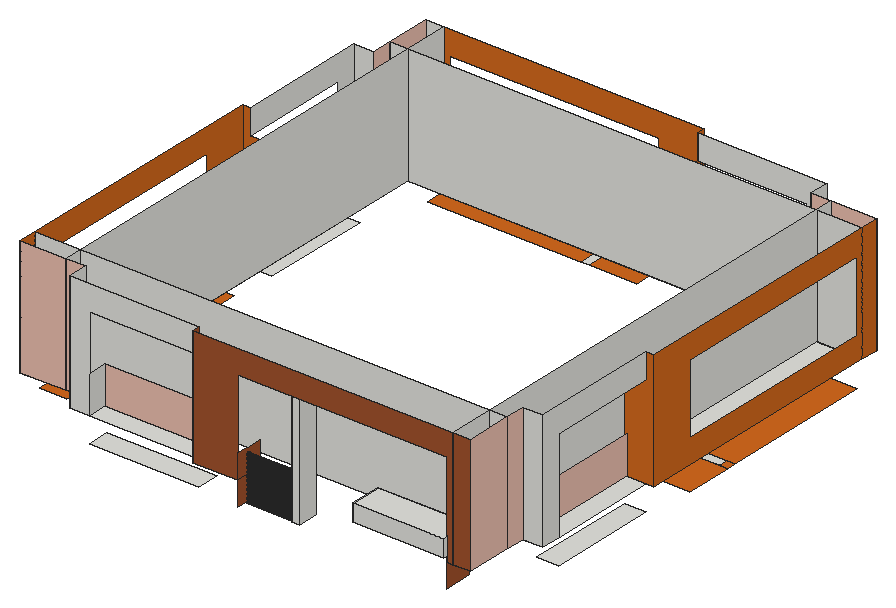
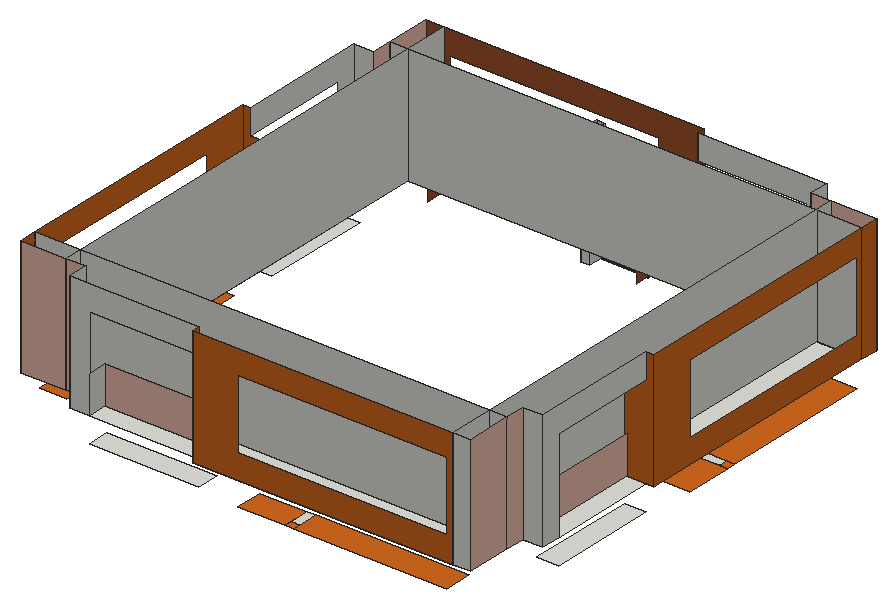
# SketchUp Ruby script. Lengths in inches.
U = 1.inch
M = Sketchup.active_model
def pt(a) = Geom::Point3d.new(a.map { |v| v * U })
def face(e, loops, mat)
  f = e.add_face(loops[0].map { |a| pt(a) })
  loops[1..].each { |l| e.add_face(l.map { |a| pt(a) }).erase! }
  f.material = f.back_material = mat if mat
  f
end
# faces: each face lists its corners as indices into pts; further lists are holes
def faces(e, pts, list, mat = nil) = list.each { |f| face(e, (f[0].is_a?(Array) ? f : [f]).map { |l| l.map { |i| pts[i] } }, mat) }
# xy, xz, yz: faces in a plane at the given z, y or x. An outline is a flat list of corners, or four numbers for a rectangle; further outlines are holes
def ring(l) = l.size == 4 ? [[l[0], l[1]], [l[2], l[1]], [l[2], l[3]], [l[0], l[3]]] : l.each_slice(2).to_a
def flat(e, list, mat, &to3) = list.each { |f| face(e, (f[0].is_a?(Array) ? f : [f]).map { |l| ring(l).map { |u, v| to3.(u, v) } }, mat) }
def xy(e, z, list, mat = nil) = flat(e, list, mat) { |x, y| [x, y, z] }
def xz(e, y, list, mat = nil) = flat(e, list, mat) { |x, z| [x, y, z] }
def yz(e, x, list, mat = nil) = flat(e, list, mat) { |y, z| [x, y, z] }
def lines(e, pts, list) = list.each { |a, b| e.add_line(pt(pts[a]), pt(pts[b])) }
# prism: a flat outline (further loops are holes) pulled along v
def prism(e, loops, v, mat = nil)
  f = face(e, loops, mat); d = Geom::Vector3d.new(v.map { |x| x * U })
  f.pushpull(f.normal.samedirection?(d) ? d.length : -d.length)
end
def box(e, o, s, mat = nil) = prism(e, [[o, [o[0] + s[0], o[1], o[2]], [o[0] + s[0], o[1] + s[1], o[2]], [o[0], o[1] + s[1], o[2]]]], [0, 0, s[2]], mat)
def at(x, y, z, deg = 0) = Geom::Transformation.translation(pt([x, y, z])) * Geom::Transformation.rotation(ORIGIN, Z_AXIS, deg.degrees)
def axes(o, x, y, z) = Geom::Transformation.new([*x, 0, *y, 0, *z, 0, *pt(o).to_a, 1])
def part(name) = M.definitions.add(name)
# library, detail: a bought-in or finely detailed component or shape, given as its bounding box
def library(name, o, s) = part(name).tap { |d| box(d.entities, o, s) }
def detail(e, o, s) = box(e.add_group.entities, o, s)
def put(e, d, t, mat = nil) = e.add_instance(d, t).tap { |i| i.material = mat if mat }
def group(e, t, mat = nil) = e.add_group.tap { |g| g.transformation = t; g.material = mat if mat }.entities
root = M.entities
M.materials.add("[0041_Chocolate]").color = [210, 105, 30]
M.materials.add("[0042_Sienna]").color = [160, 82, 45]
M.materials.add("[0119_RosyBrown]").color = [234, 190, 174]
prism(root,[[[1139,96.8125,1516.98],[1414.89,97.68,1516.98],[1415.2,0.87,1516.98],[1139.3,0,1516.98]]],[0,0,52.19])
xy(root,1422.625,[[306.65,36.8125,641.22,102.8125],[1482,271.47,1548,606.03],[72,943.59,138,1278.16],[978.78,1446.8125,1313.35,1512.8125]])
xy(root,1426.89,[[72,636.29,132,662.8],[1488,886.83,1548,913.33],[671.48,1452.8125,697.99,1512.8125]])
xy(root,1426.89,[[48,169.92,132,636.29],[48,636.29,72,662.8],[48,662.8,132,806.17],[1488,743.45,1572,886.83],[1548,886.83,1572,913.33],
  [1488,913.33,1572,1379.7],[205.11,1452.8125,671.48,1536.8125],[697.99,1452.8125,841.36,1536.8125],[671.48,1512.8125,697.99,1536.8125]],"[0041_Chocolate]")
xy(root,1500,[[1434.3125,12.8125,1488,150.5],[306.65,36.8125,641.22,96.8125],[48,96.8125,185.6875,150.5],[48,150.5,185.6875,150.5,185.6875,1399.125,132,1399.125,132,1338.16,72,1338.16,72,1278.16,132,1278.16,132,943.59,48,943.59],[1434.3125,150.5,1488,150.5,1488,211.46,1548,211.46,1548,271.47,1488,271.47,1488,606.03,1572,606.03,1572,1399.125,1434.3125,1399.125],
  [1488,271.47,1548,606.03],[72,943.59,132,1278.16],[132,1399.125,185.6875,1536.8125],[185.6875,1399.125,1434.3125,1399.125,1434.3125,1452.8125,1373.35,1452.8125,1373.35,1512.8125,1313.35,1512.8125,1313.35,1452.8125,978.78,1452.8125,978.78,1536.8125,185.6875,1536.8125],[1434.3125,1399.125,1572,1452.8125],
  [978.78,1452.8125,1313.35,1512.8125]])
xz(root,12.8125,[[641.22,1500,778.64,1500,778.64,1786.89,1414.89,1786.89,1414.89,1500,1434.3125,1500,1434.3125,1860,641.22,1860],[1434.3125,1500,1488,1860]],"[0042_Sienna]")
xz(root,36.8125,[[922.01,1426.89,948.52,1786.89],[246.65,1500,306.65,1500,306.65,1782.625,641.22,1782.625,641.22,1860,246.65,1860]])
xz(root,96.8125,[[922.01,1426.89,948.52,1786.89]])
xz(root,96.8125,[[48,1500,185.6875,1860],[185.6875,1500,246.65,1860],[306.65,1500,641.22,1613.76]],"[0119_RosyBrown]")
xz(root,150.5,[[48,1500,1488,1860]])
xz(root,211.46,[[1488,1500,1548,1860]])
xz(root,271.47,[[1488,1500,1548,1613.76]])
xz(root,606.03,[[1488,1500,1572,1500,1572,1860,1548,1860,1548,1782.625,1482,1782.625,1482,1613.76,1488,1613.76]],"[0041_Chocolate]")
xz(root,943.59,[[48,1500,48,1860,72,1860,72,1782.625,138,1782.625,138,1613.76,132,1613.76,132,1500]],"[0041_Chocolate]")
xz(root,1278.16,[[72,1500,132,1613.76]])
xz(root,1338.16,[[72,1500,132,1860]])
xz(root,1399.125,[[132,1500,1572,1860]])
xz(root,1452.8125,[[978.78,1500,1313.35,1613.76],[1373.35,1500,1434.3125,1860],[1434.3125,1500,1572,1860]],"[0119_RosyBrown]")
xz(root,1512.8125,[[1313.35,1500,1313.35,1782.625,978.78,1782.625,978.78,1860,1373.35,1860,1373.35,1500]])
xz(root,1536.8125,[[132,1500,185.6875,1860]])
xz(root,1536.8125,[[[185.6875,1500,978.78,1860],[205.11,1573.11,841.36,1786.89]]],"[0041_Chocolate]")
yz(root,48,[[96.8125,1500,150.5,1860],[[150.5,1500,943.59,1860],[169.92,1573.11,806.17,1786.89]]],"[0041_Chocolate]")
yz(root,72,[[1278.16,1500,1278.16,1782.625,943.59,1782.625,943.59,1860,1338.16,1860,1338.16,1500]])
yz(root,132,[[943.59,1500,1278.16,1613.76],[1338.16,1500,1399.125,1860],[1399.125,1500,1536.8125,1860]],"[0119_RosyBrown]")
yz(root,185.6875,[[96.8125,1500,1536.8125,1860]])
yz(root,246.65,[[36.8125,1500,96.8125,1860]])
yz(root,306.65,[[36.8125,1500,96.8125,1613.76]])
yz(root,641.22,[[12.8125,1500,12.8125,1860,36.8125,1860,36.8125,1782.625,102.8125,1782.625,102.8125,1613.76,96.8125,1613.76,96.8125,1500]],"[0042_Sienna]")
yz(root,778.64,[[48.34,1422.02,49.29,1422.14,50.18,1422.51,50.95,1423.1,51.53,1423.86,51.9,1424.75,52.03,1425.7,51.9,1426.66,51.8,1426.89,44.875,1426.89,44.78,1426.66,44.65,1425.7,44.78,1424.75,45.15,1423.86,45.73,1423.1,46.5,1422.51,47.38,1422.14]])
yz(root,778.64,[[12.8125,1426.89,44.875,1426.89,45.15,1427.55,45.73,1428.3125,46.5,1428.9,47.38,1429.27,48.34,1429.39,49.29,1429.27,50.18,1428.9,50.95,1428.3125,51.53,1427.55,51.8,1426.89,96.8125,1426.89,96.8125,1500,51.19,1500,51.53,1499.55,51.9,1498.66,52.03,1497.7,51.9,1496.75,51.53,1495.86,50.95,1495.1,50.18,1494.51,49.29,1494.14,48.34,1494.02,47.38,1494.14,46.5,1494.51,45.73,1495.1,45.15,1495.86,44.78,1496.75,44.65,1497.7,44.78,1498.66,45.15,1499.55,45.49,1500,12.8125,1500],[44.875,1426.89,51.8,1426.89,51.53,1427.55,50.95,1428.3125,50.18,1428.9,49.29,1429.27,48.34,1429.39,47.38,1429.27,46.5,1428.9,45.73,1428.3125,45.15,1427.55],[48.34,1494.02,49.29,1494.14,50.18,1494.51,50.95,1495.1,51.53,1495.86,51.9,1496.75,52.03,1497.7,51.9,1498.66,51.53,1499.55,51.19,1500,45.49,1500,45.15,1499.55,44.78,1498.66,44.65,1497.7,44.78,1496.75,45.15,1495.86,45.73,1495.1,46.5,1494.51,47.38,1494.14],[12.8125,1500,45.49,1500,45.73,1500.3125,46.5,1500.9,47.38,1501.27,48.34,1501.39,49.29,1501.27,50.18,1500.9,50.95,1500.3125,51.19,1500,96.8125,1500,96.8125,1573.11,49.67,1573.11,50.18,1572.9,50.95,1572.3125,51.53,1571.55,51.9,1570.66,52.03,1569.7,51.9,1568.75,51.53,1567.86,50.95,1567.1,50.18,1566.51,49.29,1566.14,48.34,1566.02,47.38,1566.14,46.5,1566.51,45.73,1567.1,45.15,1567.86,44.78,1568.75,44.65,1569.7,44.78,1570.66,45.15,1571.55,45.73,1572.3125,46.5,1572.9,47.01,1573.11,12.8125,1573.11],[45.49,1500,51.19,1500,50.95,1500.3125,50.18,1500.9,49.29,1501.27,48.34,1501.39,47.38,1501.27,46.5,1500.9,45.73,1500.3125]],"[0042_Sienna]")
yz(root,922.01,[[48.34,1422.02,47.38,1422.14,46.5,1422.51,45.73,1423.1,45.15,1423.86,44.78,1424.75,44.65,1425.7,44.78,1426.66,44.875,1426.89,51.8,1426.89,51.9,1426.66,52.03,1425.7,51.9,1424.75,51.53,1423.86,50.95,1423.1,50.18,1422.51,49.29,1422.14],[[36.8125,1426.89,36.8125,1786.89,96.8125,1786.89,96.8125,1426.89,51.8,1426.89,51.53,1427.55,50.95,1428.3125,50.18,1428.9,49.29,1429.27,48.34,1429.39,47.38,1429.27,46.5,1428.9,45.73,1428.3125,45.15,1427.55,44.875,1426.89],[48.34,1578.02,49.29,1578.14,50.18,1578.51,50.95,1579.1,51.53,1579.86,51.9,1580.75,52.03,1581.7,51.9,1582.66,51.53,1583.55,50.95,1584.3125,50.18,1584.9,49.29,1585.27,48.34,1585.39,47.38,1585.27,46.5,1584.9,45.73,1584.3125,45.15,1583.55,44.78,1582.66,44.65,1581.7,44.78,1580.75,45.15,1579.86,45.73,1579.1,46.5,1578.51,47.38,1578.14]],[44.875,1426.89,45.15,1427.55,45.73,1428.3125,46.5,1428.9,47.38,1429.27,48.34,1429.39,49.29,1429.27,50.18,1428.9,50.95,1428.3125,51.53,1427.55,51.8,1426.89]])
yz(root,948.52,[[36.8125,1426.89,96.8125,1786.89]])
yz(root,978.78,[[1452.8125,1500,1536.8125,1500,1536.8125,1860,1512.8125,1860,1512.8125,1782.625,1446.8125,1782.625,1446.8125,1613.76,1452.8125,1613.76]],"[0041_Chocolate]")
yz(root,1313.35,[[1452.8125,1500,1512.8125,1613.76]])
yz(root,1373.35,[[1452.8125,1500,1512.8125,1860]])
yz(root,1414.89,[[12.8125,1426.89,96.8125,1500],[12.8125,1500,96.8125,1573.11]],"[0042_Sienna]")
yz(root,1434.3125,[[12.8125,1500,1452.8125,1860]])
yz(root,1488,[[12.8125,1500,150.5,1860],[150.5,1500,211.46,1860],[271.47,1500,606.03,1613.76]],"[0119_RosyBrown]")
yz(root,1548,[[211.46,1500,271.47,1500,271.47,1782.625,606.03,1782.625,606.03,1860,211.46,1860]])
yz(root,1572,[[[606.03,1500,1399.125,1860],[743.45,1573.11,1379.7,1786.89]],[1399.125,1500,1452.8125,1860]],"[0041_Chocolate]")
p = [[922.01,48.34,1422.02],[922.01,47.38,1422.14],[778.64,47.38,1422.14],[778.64,48.34,1422.02],[922.01,49.29,1422.14],[778.64,49.29,1422.14],
  [922.01,46.5,1422.51],[778.64,46.5,1422.51],[922.01,50.18,1422.51],[778.64,50.18,1422.51],[922.01,45.73,1423.1],[778.64,45.73,1423.1],
  [922.01,50.95,1423.1],[778.64,50.95,1423.1],[922.01,45.15,1423.86],[778.64,45.15,1423.86],[922.01,51.53,1423.86],[778.64,51.53,1423.86],
  [922.01,44.78,1424.75],[778.64,44.78,1424.75],[922.01,51.9,1424.75],[778.64,51.9,1424.75],[922.01,44.65,1425.7],[778.64,44.65,1425.7],
  [922.01,52.03,1425.7],[778.64,52.03,1425.7],[922.01,44.78,1426.66],[778.64,44.78,1426.66],[922.01,51.9,1426.66],[778.64,51.9,1426.66],
  [922.01,44.875,1426.89],[922.01,45.15,1427.55],[778.64,45.15,1427.55],[778.64,44.875,1426.89],[922.01,51.53,1427.55],[922.01,51.8,1426.89],
  [778.64,51.8,1426.89],[778.64,51.53,1427.55],[922.01,45.73,1428.3125],[778.64,45.73,1428.3125],[922.01,50.95,1428.3125],[778.64,50.95,1428.3125],
  [922.01,46.5,1428.9],[778.64,46.5,1428.9],[922.01,50.18,1428.9],[778.64,50.18,1428.9],[922.01,47.38,1429.27],[778.64,47.38,1429.27],
  [922.01,49.29,1429.27],[778.64,49.29,1429.27],[922.01,48.34,1429.39],[778.64,48.34,1429.39],[922.01,48.34,1434.02],[922.01,47.38,1434.14],
  [778.64,47.38,1434.14],[778.64,48.34,1434.02],[922.01,49.29,1434.14],[778.64,49.29,1434.14],[922.01,46.5,1434.51],[778.64,46.5,1434.51],
  [922.01,50.18,1434.51],[778.64,50.18,1434.51],[922.01,45.73,1435.1],[778.64,45.73,1435.1],[922.01,50.95,1435.1],[778.64,50.95,1435.1],
  [922.01,45.15,1435.86],[778.64,45.15,1435.86],[922.01,51.53,1435.86],[778.64,51.53,1435.86],[922.01,44.78,1436.75],[778.64,44.78,1436.75],
  [922.01,51.9,1436.75],[778.64,51.9,1436.75],[922.01,44.65,1437.7],[778.64,44.65,1437.7],[922.01,52.03,1437.7],[778.64,52.03,1437.7],
  [922.01,44.78,1438.66],[778.64,44.78,1438.66],[922.01,51.9,1438.66],[778.64,51.9,1438.66],[922.01,45.15,1439.55],[778.64,45.15,1439.55],
  [922.01,51.53,1439.55],[778.64,51.53,1439.55],[922.01,45.73,1440.3125],[778.64,45.73,1440.3125],[922.01,50.95,1440.3125],[778.64,50.95,1440.3125],
  [922.01,46.5,1440.9],[778.64,46.5,1440.9],[922.01,50.18,1440.9],[778.64,50.18,1440.9],[922.01,47.38,1441.27],[778.64,47.38,1441.27],
  [922.01,49.29,1441.27],[778.64,49.29,1441.27],[922.01,48.34,1441.39],[778.64,48.34,1441.39],[922.01,48.34,1446.02],[922.01,47.38,1446.14],
  [778.64,47.38,1446.14],[778.64,48.34,1446.02],[922.01,49.29,1446.14],[778.64,49.29,1446.14],[922.01,46.5,1446.51],[778.64,46.5,1446.51],
  [922.01,50.18,1446.51],[778.64,50.18,1446.51],[922.01,45.73,1447.1],[778.64,45.73,1447.1],[922.01,50.95,1447.1],[778.64,50.95,1447.1],
  [922.01,45.15,1447.86],[778.64,45.15,1447.86],[922.01,51.53,1447.86],[778.64,51.53,1447.86],[922.01,44.78,1448.75],[778.64,44.78,1448.75],
  [922.01,51.9,1448.75],[778.64,51.9,1448.75],[922.01,44.65,1449.7],[778.64,44.65,1449.7],[922.01,52.03,1449.7],[778.64,52.03,1449.7],
  [922.01,44.78,1450.66],[778.64,44.78,1450.66],[922.01,51.9,1450.66],[778.64,51.9,1450.66],[922.01,45.15,1451.55],[778.64,45.15,1451.55],
  [922.01,51.53,1451.55],[778.64,51.53,1451.55],[922.01,45.73,1452.3125],[778.64,45.73,1452.3125],[922.01,50.95,1452.3125],[778.64,50.95,1452.3125],
  [922.01,46.5,1452.9],[778.64,46.5,1452.9],[922.01,50.18,1452.9],[778.64,50.18,1452.9],[922.01,47.38,1453.27],[778.64,47.38,1453.27],
  [922.01,49.29,1453.27],[778.64,49.29,1453.27],[922.01,48.34,1453.39],[778.64,48.34,1453.39],[922.01,48.34,1458.02],[922.01,47.38,1458.14],
  [778.64,47.38,1458.14],[778.64,48.34,1458.02],[922.01,49.29,1458.14],[778.64,49.29,1458.14],[922.01,46.5,1458.51],[778.64,46.5,1458.51],
  [922.01,50.18,1458.51],[778.64,50.18,1458.51],[922.01,45.73,1459.1],[778.64,45.73,1459.1],[922.01,50.95,1459.1],[778.64,50.95,1459.1],
  [922.01,45.15,1459.86],[778.64,45.15,1459.86],[922.01,51.53,1459.86],[778.64,51.53,1459.86],[922.01,44.78,1460.75],[778.64,44.78,1460.75],
  [922.01,51.9,1460.75],[778.64,51.9,1460.75],[922.01,44.65,1461.7],[778.64,44.65,1461.7],[922.01,52.03,1461.7],[778.64,52.03,1461.7],
  [922.01,44.78,1462.66],[778.64,44.78,1462.66],[922.01,51.9,1462.66],[778.64,51.9,1462.66],[922.01,45.15,1463.55],[778.64,45.15,1463.55],
  [922.01,51.53,1463.55],[778.64,51.53,1463.55],[922.01,45.73,1464.3125],[778.64,45.73,1464.3125],[922.01,50.95,1464.3125],[778.64,50.95,1464.3125],
  [922.01,46.5,1464.9],[778.64,46.5,1464.9],[922.01,50.18,1464.9],[778.64,50.18,1464.9],[922.01,47.38,1465.27],[778.64,47.38,1465.27],
  [922.01,49.29,1465.27],[778.64,49.29,1465.27],[922.01,48.34,1465.39],[778.64,48.34,1465.39],[922.01,48.34,1470.02],[922.01,47.38,1470.14],
  [778.64,47.38,1470.14],[778.64,48.34,1470.02],[922.01,49.29,1470.14],[778.64,49.29,1470.14],[922.01,46.5,1470.51],[778.64,46.5,1470.51],
  [922.01,50.18,1470.51],[778.64,50.18,1470.51],[922.01,45.73,1471.1],[778.64,45.73,1471.1],[922.01,50.95,1471.1],[778.64,50.95,1471.1],
  [922.01,45.15,1471.86],[778.64,45.15,1471.86],[922.01,51.53,1471.86],[778.64,51.53,1471.86],[922.01,44.78,1472.75],[778.64,44.78,1472.75],
  [922.01,51.9,1472.75],[778.64,51.9,1472.75],[922.01,44.65,1473.7],[778.64,44.65,1473.7],[922.01,52.03,1473.7],[778.64,52.03,1473.7],
  [922.01,44.78,1474.66],[778.64,44.78,1474.66],[922.01,51.9,1474.66],[778.64,51.9,1474.66],[922.01,45.15,1475.55],[778.64,45.15,1475.55],
  [922.01,51.53,1475.55],[778.64,51.53,1475.55],[922.01,45.73,1476.3125],[778.64,45.73,1476.3125],[922.01,50.95,1476.3125],[778.64,50.95,1476.3125],
  [922.01,46.5,1476.9],[778.64,46.5,1476.9],[922.01,50.18,1476.9],[778.64,50.18,1476.9],[922.01,47.38,1477.27],[778.64,47.38,1477.27],
  [922.01,49.29,1477.27],[778.64,49.29,1477.27],[922.01,48.34,1477.39],[778.64,48.34,1477.39],[922.01,48.34,1482.02],[922.01,47.38,1482.14],
  [778.64,47.38,1482.14],[778.64,48.34,1482.02],[922.01,49.29,1482.14],[778.64,49.29,1482.14],[922.01,46.5,1482.51],[778.64,46.5,1482.51],
  [922.01,50.18,1482.51],[778.64,50.18,1482.51],[922.01,45.73,1483.1],[778.64,45.73,1483.1],[922.01,50.95,1483.1],[778.64,50.95,1483.1],
  [922.01,45.15,1483.86],[778.64,45.15,1483.86],[922.01,51.53,1483.86],[778.64,51.53,1483.86],[922.01,44.78,1484.75],[778.64,44.78,1484.75],
  [922.01,51.9,1484.75],[778.64,51.9,1484.75],[922.01,44.65,1485.7],[778.64,44.65,1485.7],[922.01,52.03,1485.7],[778.64,52.03,1485.7],
  [922.01,44.78,1486.66],[778.64,44.78,1486.66],[922.01,51.9,1486.66],[778.64,51.9,1486.66],[922.01,45.15,1487.55],[778.64,45.15,1487.55],
  [922.01,51.53,1487.55],[778.64,51.53,1487.55],[922.01,45.73,1488.3125],[778.64,45.73,1488.3125],[922.01,50.95,1488.3125],[778.64,50.95,1488.3125],
  [922.01,46.5,1488.9],[778.64,46.5,1488.9],[922.01,50.18,1488.9],[778.64,50.18,1488.9],[922.01,47.38,1489.27],[778.64,47.38,1489.27],
  [922.01,49.29,1489.27],[778.64,49.29,1489.27],[922.01,48.34,1489.39],[778.64,48.34,1489.39],[922.01,48.34,1494.02],[922.01,47.38,1494.14],
  [778.64,47.38,1494.14],[778.64,48.34,1494.02],[922.01,49.29,1494.14],[778.64,49.29,1494.14],[922.01,46.5,1494.51],[778.64,46.5,1494.51],
  [922.01,50.18,1494.51],[778.64,50.18,1494.51],[922.01,45.73,1495.1],[778.64,45.73,1495.1],[922.01,50.95,1495.1],[778.64,50.95,1495.1],
  [922.01,45.15,1495.86],[778.64,45.15,1495.86],[922.01,51.53,1495.86],[778.64,51.53,1495.86],[922.01,44.78,1496.75],[778.64,44.78,1496.75],
  [922.01,51.9,1496.75],[778.64,51.9,1496.75],[922.01,44.65,1497.7],[778.64,44.65,1497.7],[922.01,52.03,1497.7],[778.64,52.03,1497.7],
  [922.01,44.78,1498.66],[778.64,44.78,1498.66],[922.01,51.9,1498.66],[778.64,51.9,1498.66],[922.01,45.15,1499.55],[778.64,45.15,1499.55],
  [922.01,51.53,1499.55],[778.64,51.53,1499.55],[922.01,45.73,1500.3125],[778.64,45.73,1500.3125],[778.64,45.49,1500],[922.01,50.95,1500.3125],
  [778.64,51.19,1500],[778.64,50.95,1500.3125],[922.01,46.5,1500.9],[778.64,46.5,1500.9],[922.01,50.18,1500.9],[778.64,50.18,1500.9],
  [922.01,47.38,1501.27],[778.64,47.38,1501.27],[922.01,49.29,1501.27],[778.64,49.29,1501.27],[922.01,48.34,1501.39],[778.64,48.34,1501.39],
  [922.01,48.34,1506.02],[922.01,47.38,1506.14],[778.64,47.38,1506.14],[778.64,48.34,1506.02],[922.01,49.29,1506.14],[778.64,49.29,1506.14],
  [922.01,46.5,1506.51],[778.64,46.5,1506.51],[922.01,50.18,1506.51],[778.64,50.18,1506.51],[922.01,45.73,1507.1],[778.64,45.73,1507.1],
  [922.01,50.95,1507.1],[778.64,50.95,1507.1],[922.01,45.15,1507.86],[778.64,45.15,1507.86],[922.01,51.53,1507.86],[778.64,51.53,1507.86],
  [922.01,44.78,1508.75],[778.64,44.78,1508.75],[922.01,51.9,1508.75],[778.64,51.9,1508.75],[922.01,44.65,1509.7],[778.64,44.65,1509.7],
  [922.01,52.03,1509.7],[778.64,52.03,1509.7],[922.01,44.78,1510.66],[778.64,44.78,1510.66],[922.01,51.9,1510.66],[778.64,51.9,1510.66],
  [922.01,45.15,1511.55],[778.64,45.15,1511.55],[922.01,51.53,1511.55],[778.64,51.53,1511.55],[922.01,45.73,1512.3125],[778.64,45.73,1512.3125],
  [922.01,50.95,1512.3125],[778.64,50.95,1512.3125],[922.01,46.5,1512.9],[778.64,46.5,1512.9],[922.01,50.18,1512.9],[778.64,50.18,1512.9],
  [922.01,47.38,1513.27],[778.64,47.38,1513.27],[922.01,49.29,1513.27],[778.64,49.29,1513.27],[922.01,48.34,1513.39],[778.64,48.34,1513.39],
  [922.01,48.34,1518.02],[922.01,47.38,1518.14],[778.64,47.38,1518.14],[778.64,48.34,1518.02],[922.01,49.29,1518.14],[778.64,49.29,1518.14],
  [922.01,46.5,1518.51],[778.64,46.5,1518.51],[922.01,50.18,1518.51],[778.64,50.18,1518.51],[922.01,45.73,1519.1],[778.64,45.73,1519.1],
  [922.01,50.95,1519.1],[778.64,50.95,1519.1],[922.01,45.15,1519.86],[778.64,45.15,1519.86],[922.01,51.53,1519.86],[778.64,51.53,1519.86],
  [922.01,44.78,1520.75],[778.64,44.78,1520.75],[922.01,51.9,1520.75],[778.64,51.9,1520.75],[922.01,44.65,1521.7],[778.64,44.65,1521.7],
  [922.01,52.03,1521.7],[778.64,52.03,1521.7],[922.01,44.78,1522.66],[778.64,44.78,1522.66],[922.01,51.9,1522.66],[778.64,51.9,1522.66],
  [922.01,45.15,1523.55],[778.64,45.15,1523.55],[922.01,51.53,1523.55],[778.64,51.53,1523.55],[922.01,45.73,1524.3125],[778.64,45.73,1524.3125],
  [922.01,50.95,1524.3125],[778.64,50.95,1524.3125],[922.01,46.5,1524.9],[778.64,46.5,1524.9],[922.01,50.18,1524.9],[778.64,50.18,1524.9],
  [922.01,47.38,1525.27],[778.64,47.38,1525.27],[922.01,49.29,1525.27],[778.64,49.29,1525.27],[922.01,48.34,1525.39],[778.64,48.34,1525.39],
  [922.01,48.34,1530.02],[922.01,47.38,1530.14],[778.64,47.38,1530.14],[778.64,48.34,1530.02],[922.01,49.29,1530.14],[778.64,49.29,1530.14],
  [922.01,46.5,1530.51],[778.64,46.5,1530.51],[922.01,50.18,1530.51],[778.64,50.18,1530.51],[922.01,45.73,1531.1],[778.64,45.73,1531.1],
  [922.01,50.95,1531.1],[778.64,50.95,1531.1],[922.01,45.15,1531.86],[778.64,45.15,1531.86],[922.01,51.53,1531.86],[778.64,51.53,1531.86],
  [922.01,44.78,1532.75],[778.64,44.78,1532.75],[922.01,51.9,1532.75],[778.64,51.9,1532.75],[922.01,44.65,1533.7],[778.64,44.65,1533.7],
  [922.01,52.03,1533.7],[778.64,52.03,1533.7],[922.01,44.78,1534.66],[778.64,44.78,1534.66],[922.01,51.9,1534.66],[778.64,51.9,1534.66],
  [922.01,45.15,1535.55],[778.64,45.15,1535.55],[922.01,51.53,1535.55],[778.64,51.53,1535.55],[922.01,45.73,1536.3125],[778.64,45.73,1536.3125],
  [922.01,50.95,1536.3125],[778.64,50.95,1536.3125],[922.01,46.5,1536.9],[778.64,46.5,1536.9],[922.01,50.18,1536.9],[778.64,50.18,1536.9],
  [922.01,47.38,1537.27],[778.64,47.38,1537.27],[922.01,49.29,1537.27],[778.64,49.29,1537.27],[922.01,48.34,1537.39],[778.64,48.34,1537.39],
  [922.01,48.34,1542.02],[922.01,47.38,1542.14],[778.64,47.38,1542.14],[778.64,48.34,1542.02],[922.01,49.29,1542.14],[778.64,49.29,1542.14],
  [922.01,46.5,1542.51],[778.64,46.5,1542.51],[922.01,50.18,1542.51],[778.64,50.18,1542.51],[922.01,45.73,1543.1],[778.64,45.73,1543.1],
  [922.01,50.95,1543.1],[778.64,50.95,1543.1],[922.01,45.15,1543.86],[778.64,45.15,1543.86],[922.01,51.53,1543.86],[778.64,51.53,1543.86],
  [922.01,44.78,1544.75],[778.64,44.78,1544.75],[922.01,51.9,1544.75],[778.64,51.9,1544.75],[922.01,44.65,1545.7],[778.64,44.65,1545.7],
  [922.01,52.03,1545.7],[778.64,52.03,1545.7],[922.01,44.78,1546.66],[778.64,44.78,1546.66],[922.01,51.9,1546.66],[778.64,51.9,1546.66],
  [922.01,45.15,1547.55],[778.64,45.15,1547.55],[922.01,51.53,1547.55],[778.64,51.53,1547.55],[922.01,45.73,1548.3125],[778.64,45.73,1548.3125],
  [922.01,50.95,1548.3125],[778.64,50.95,1548.3125],[922.01,46.5,1548.9],[778.64,46.5,1548.9],[922.01,50.18,1548.9],[778.64,50.18,1548.9],
  [922.01,47.38,1549.27],[778.64,47.38,1549.27],[922.01,49.29,1549.27],[778.64,49.29,1549.27],[922.01,48.34,1549.39],[778.64,48.34,1549.39],
  [922.01,48.34,1554.02],[922.01,47.38,1554.14],[778.64,47.38,1554.14],[778.64,48.34,1554.02],[922.01,49.29,1554.14],[778.64,49.29,1554.14],
  [922.01,46.5,1554.51],[778.64,46.5,1554.51],[922.01,50.18,1554.51],[778.64,50.18,1554.51],[922.01,45.73,1555.1],[778.64,45.73,1555.1],
  [922.01,50.95,1555.1],[778.64,50.95,1555.1],[922.01,45.15,1555.86],[778.64,45.15,1555.86],[922.01,51.53,1555.86],[778.64,51.53,1555.86],
  [922.01,44.78,1556.75],[778.64,44.78,1556.75],[922.01,51.9,1556.75],[778.64,51.9,1556.75],[922.01,44.65,1557.7],[778.64,44.65,1557.7],
  [922.01,52.03,1557.7],[778.64,52.03,1557.7],[922.01,44.78,1558.66],[778.64,44.78,1558.66],[922.01,51.9,1558.66],[778.64,51.9,1558.66],
  [922.01,45.15,1559.55],[778.64,45.15,1559.55],[922.01,51.53,1559.55],[778.64,51.53,1559.55],[922.01,45.73,1560.3125],[778.64,45.73,1560.3125],
  [922.01,50.95,1560.3125],[778.64,50.95,1560.3125],[922.01,46.5,1560.9],[778.64,46.5,1560.9],[922.01,50.18,1560.9],[778.64,50.18,1560.9],
  [922.01,47.38,1561.27],[778.64,47.38,1561.27],[922.01,49.29,1561.27],[778.64,49.29,1561.27],[922.01,48.34,1561.39],[778.64,48.34,1561.39]]
faces(root,p,[[0,1,2,3],[4,0,3,5],[1,6,7,2],[8,4,5,9],[6,10,11,7],[12,8,9,13],[10,14,15,11],[16,12,13,17],
  [14,18,19,15],[20,16,17,21],[18,22,23,19],[24,20,21,25],[22,26,27,23],[28,24,25,29],[26,30,31,32,33,27],[34,35,28,29,36,37],
  [31,38,39,32],[40,34,37,41],[38,42,43,39],[44,40,41,45],[42,46,47,43],[48,44,45,49],[46,50,51,47],[50,48,49,51],
  [52,53,54,55],[56,52,55,57],[53,58,59,54],[60,56,57,61],[58,62,63,59],[64,60,61,65],[62,66,67,63],[68,64,65,69],
  [66,70,71,67],[72,68,69,73],[70,74,75,71],[76,72,73,77],[74,78,79,75],[80,76,77,81],[78,82,83,79],[84,80,81,85],
  [82,86,87,83],[88,84,85,89],[86,90,91,87],[92,88,89,93],[90,94,95,91],[96,92,93,97],[94,98,99,95],[98,96,97,99],
  [100,101,102,103],[104,100,103,105],[101,106,107,102],[108,104,105,109],[106,110,111,107],[112,108,109,113],[110,114,115,111],[116,112,113,117],
  [114,118,119,115],[120,116,117,121],[118,122,123,119],[124,120,121,125],[122,126,127,123],[128,124,125,129],[126,130,131,127],[132,128,129,133],
  [130,134,135,131],[136,132,133,137],[134,138,139,135],[140,136,137,141],[138,142,143,139],[144,140,141,145],[142,146,147,143],[146,144,145,147],
  [148,149,150,151],[152,148,151,153],[149,154,155,150],[156,152,153,157],[154,158,159,155],[160,156,157,161],[158,162,163,159],[164,160,161,165],
  [162,166,167,163],[168,164,165,169],[166,170,171,167],[172,168,169,173],[170,174,175,171],[176,172,173,177],[174,178,179,175],[180,176,177,181],
  [178,182,183,179],[184,180,181,185],[182,186,187,183],[188,184,185,189],[186,190,191,187],[192,188,189,193],[190,194,195,191],[194,192,193,195],
  [196,197,198,199],[200,196,199,201],[197,202,203,198],[204,200,201,205],[202,206,207,203],[208,204,205,209],[206,210,211,207],[212,208,209,213],
  [210,214,215,211],[216,212,213,217],[214,218,219,215],[220,216,217,221],[218,222,223,219],[224,220,221,225],[222,226,227,223],[228,224,225,229],
  [226,230,231,227],[232,228,229,233],[230,234,235,231],[236,232,233,237],[234,238,239,235],[240,236,237,241],[238,242,243,239],[242,240,241,243],
  [244,245,246,247],[248,244,247,249],[245,250,251,246],[252,248,249,253],[250,254,255,251],[256,252,253,257],[254,258,259,255],[260,256,257,261],
  [258,262,263,259],[264,260,261,265],[262,266,267,263],[268,264,265,269],[266,270,271,267],[272,268,269,273],[270,274,275,271],[276,272,273,277],
  [274,278,279,275],[280,276,277,281],[278,282,283,279],[284,280,281,285],[282,286,287,283],[288,284,285,289],[286,290,291,287],[290,288,289,291],
  [292,293,294,295],[296,292,295,297],[293,298,299,294],[300,296,297,301],[298,302,303,299],[304,300,301,305],[302,306,307,303],[308,304,305,309],
  [306,310,311,307],[312,308,309,313],[310,314,315,311],[316,312,313,317],[314,318,319,315],[320,316,317,321],[318,322,323,319],[324,320,321,325],
  [322,326,327,328,323],[329,324,325,330,331],[326,332,333,327],[334,329,331,335],[332,336,337,333],[338,334,335,339],[336,340,341,337],[340,338,339,341],
  [342,343,344,345],[346,342,345,347],[343,348,349,344],[350,346,347,351],[348,352,353,349],[354,350,351,355],[352,356,357,353],[358,354,355,359],
  [356,360,361,357],[362,358,359,363],[360,364,365,361],[366,362,363,367],[364,368,369,365],[370,366,367,371],[368,372,373,369],[374,370,371,375],
  [372,376,377,373],[378,374,375,379],[376,380,381,377],[382,378,379,383],[380,384,385,381],[386,382,383,387],[384,388,389,385],[388,386,387,389],
  [390,391,392,393],[394,390,393,395],[391,396,397,392],[398,394,395,399],[396,400,401,397],[402,398,399,403],[400,404,405,401],[406,402,403,407],
  [404,408,409,405],[410,406,407,411],[408,412,413,409],[414,410,411,415],[412,416,417,413],[418,414,415,419],[416,420,421,417],[422,418,419,423],
  [420,424,425,421],[426,422,423,427],[424,428,429,425],[430,426,427,431],[428,432,433,429],[434,430,431,435],[432,436,437,433],[436,434,435,437],
  [438,439,440,441],[442,438,441,443],[439,444,445,440],[446,442,443,447],[444,448,449,445],[450,446,447,451],[448,452,453,449],[454,450,451,455],
  [452,456,457,453],[458,454,455,459],[456,460,461,457],[462,458,459,463],[460,464,465,461],[466,462,463,467],[464,468,469,465],[470,466,467,471],
  [468,472,473,469],[474,470,471,475],[472,476,477,473],[478,474,475,479],[476,480,481,477],[482,478,479,483],[480,484,485,481],[484,482,483,485],
  [486,487,488,489],[490,486,489,491],[487,492,493,488],[494,490,491,495],[492,496,497,493],[498,494,495,499],[496,500,501,497],[502,498,499,503],
  [500,504,505,501],[506,502,503,507],[504,508,509,505],[510,506,507,511],[508,512,513,509],[514,510,511,515],[512,516,517,513],[518,514,515,519],
  [516,520,521,517],[522,518,519,523],[520,524,525,521],[526,522,523,527],[524,528,529,525],[530,526,527,531],[528,532,533,529],[532,530,531,533],
  [534,535,536,537],[538,534,537,539],[535,540,541,536],[542,538,539,543],[540,544,545,541],[546,542,543,547],[544,548,549,545],[550,546,547,551],
  [548,552,553,549],[554,550,551,555],[552,556,557,553],[558,554,555,559],[556,560,561,557],[562,558,559,563],[560,564,565,561],[566,562,563,567],
  [564,568,569,565],[570,566,567,571],[568,572,573,569],[574,570,571,575],[572,576,577,573],[578,574,575,579],[576,580,581,577],[580,578,579,581]])
